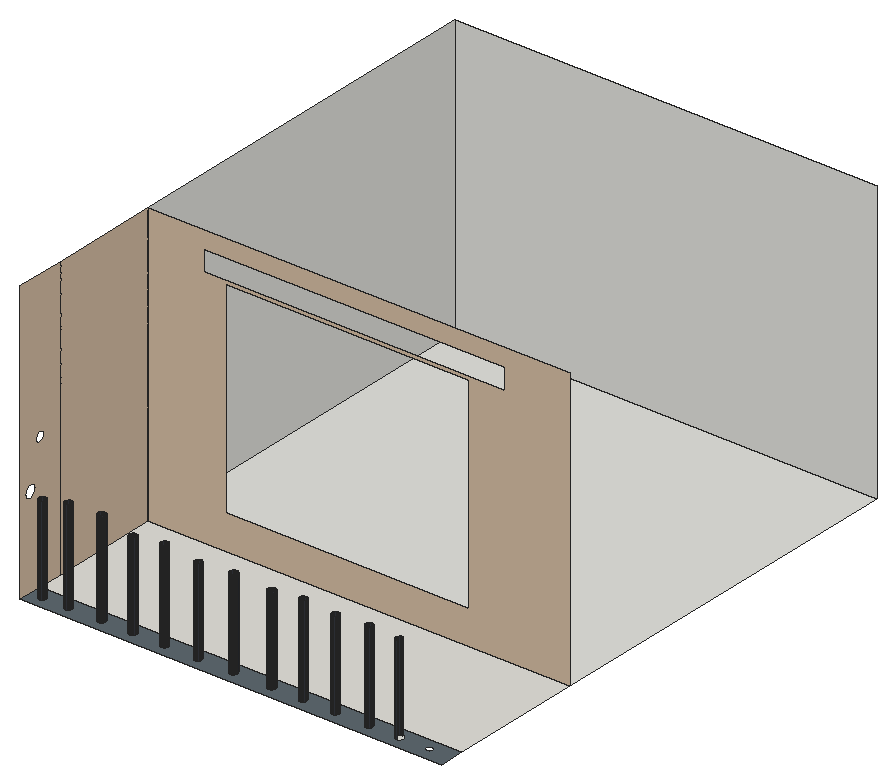
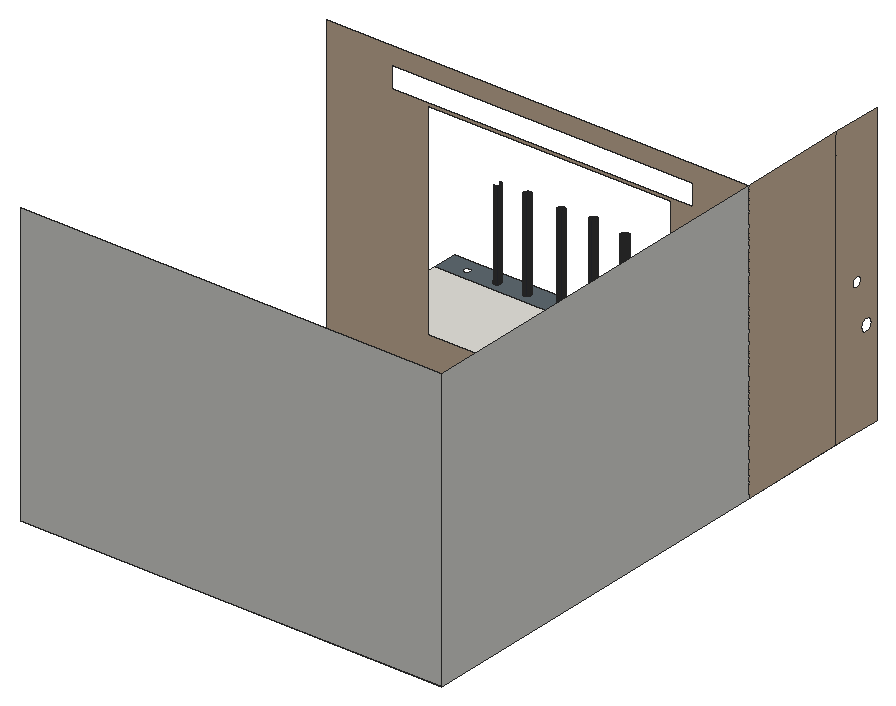
# SketchUp Ruby script. Lengths in inches.
U = 1.inch
M = Sketchup.active_model
def pt(a) = Geom::Point3d.new(a.map { |v| v * U })
def face(e, loops, mat)
  f = e.add_face(loops[0].map { |a| pt(a) })
  loops[1..].each { |l| e.add_face(l.map { |a| pt(a) }).erase! }
  f.material = f.back_material = mat if mat
  f
end
# faces: each face lists its corners as indices into pts; further lists are holes
def faces(e, pts, list, mat = nil) = list.each { |f| face(e, (f[0].is_a?(Array) ? f : [f]).map { |l| l.map { |i| pts[i] } }, mat) }
# xy, xz, yz: faces in a plane at the given z, y or x. An outline is a flat list of corners, or four numbers for a rectangle; further outlines are holes
def ring(l) = l.size == 4 ? [[l[0], l[1]], [l[2], l[1]], [l[2], l[3]], [l[0], l[3]]] : l.each_slice(2).to_a
def flat(e, list, mat, &to3) = list.each { |f| face(e, (f[0].is_a?(Array) ? f : [f]).map { |l| ring(l).map { |u, v| to3.(u, v) } }, mat) }
def xy(e, z, list, mat = nil) = flat(e, list, mat) { |x, y| [x, y, z] }
def xz(e, y, list, mat = nil) = flat(e, list, mat) { |x, z| [x, y, z] }
def yz(e, x, list, mat = nil) = flat(e, list, mat) { |y, z| [x, y, z] }
def lines(e, pts, list) = list.each { |a, b| e.add_line(pt(pts[a]), pt(pts[b])) }
# prism: a flat outline (further loops are holes) pulled along v
def prism(e, loops, v, mat = nil)
  f = face(e, loops, mat); d = Geom::Vector3d.new(v.map { |x| x * U })
  f.pushpull(f.normal.samedirection?(d) ? d.length : -d.length)
end
def box(e, o, s, mat = nil) = prism(e, [[o, [o[0] + s[0], o[1], o[2]], [o[0] + s[0], o[1] + s[1], o[2]], [o[0], o[1] + s[1], o[2]]]], [0, 0, s[2]], mat)
def at(x, y, z, deg = 0) = Geom::Transformation.translation(pt([x, y, z])) * Geom::Transformation.rotation(ORIGIN, Z_AXIS, deg.degrees)
def axes(o, x, y, z) = Geom::Transformation.new([*x, 0, *y, 0, *z, 0, *pt(o).to_a, 1])
def part(name) = M.definitions.add(name)
# library, detail: a bought-in or finely detailed component or shape, given as its bounding box
def library(name, o, s) = part(name).tap { |d| box(d.entities, o, s) }
def detail(e, o, s) = box(e.add_group.entities, o, s)
def put(e, d, t, mat = nil) = e.add_instance(d, t).tap { |i| i.material = mat if mat }
def group(e, t, mat = nil) = e.add_group.tap { |g| g.transformation = t; g.material = mat if mat }.entities
root = M.entities
M.materials.add("[Formica Laminate Dark]").color = [50, 53, 60]
M.materials.add("[Formica Laminate Light]").color = [213, 189, 164]
M.materials.add("[Formica Speckled Grey]").color = [94, 105, 111]
M.materials.add("[Marble Carrara Gold Floor Tile]").color = [225, 223, 217]
xy(root,381,[[13.88,126.78,13.48,126.87,13.125,127.0625,12.83,127.34,12.61,127.6875,12.49,128.08,12.48,128.48,12.57,128.88,12.76,129.24,13.04,129.54,13.39,129.76,13.78,129.875,14.18,129.89,14.58,129.8,14.94,129.6,15.24,129.33,15.46,128.98,15.57,128.59,15.59,128.18,15.5,127.78,15.3,127.42,15.03,127.125,14.68,126.91,14.29,126.79],[25.07,126.78,24.67,126.87,24.3125,127.0625,24.01,127.34,23.8,127.6875,23.68,128.08,23.67,128.48,23.76,128.88,23.95,129.24,24.23,129.54,24.57,129.76,24.96,129.875,25.37,129.89,25.77,129.8,26.13,129.6,26.43,129.33,26.64,128.98,26.76,128.59,26.78,128.18,26.68,127.78,26.49,127.42,26.21,127.125,25.87,126.91,25.48,126.79],[39.26,126.78,38.86,126.87,38.5,127.0625,38.2,127.34,37.99,127.6875,37.87,128.08,37.85,128.48,37.94,128.88,38.14,129.24,38.42,129.54,38.76,129.76,39.15,129.875,39.56,129.89,39.96,129.8,40.32,129.6,40.61,129.33,40.83,128.98,40.95,128.59,40.96,128.18,40.87,127.78,40.68,127.42,40.4,127.125,40.05,126.91,39.66,126.79],[52.63,126.78,52.23,126.87,51.875,127.0625,51.58,127.34,51.36,127.6875,51.24,128.08,51.23,128.48,51.32,128.88,51.51,129.24,51.79,129.54,52.14,129.76,52.53,129.875,52.93,129.89,53.33,129.8,53.69,129.6,53.99,129.33,54.21,128.98,54.32,128.59,54.34,128.18,54.25,127.78,54.05,127.42,53.78,127.125,53.43,126.91,53.04,126.79],[66.19,126.78,65.8,126.87,65.4375,127.0625,65.14,127.34,64.92,127.6875,64.8,128.08,64.79,128.48,64.88,128.88,65.07,129.24,65.35,129.54,65.7,129.76,66.09,129.875,66.5,129.89,66.89,129.8,67.25,129.6,67.55,129.33,67.77,128.98,67.89,128.59,67.9,128.18,67.81,127.78,67.62,127.42,67.34,127.125,66.99,126.91,66.6,126.79],
  [80.57,126.78,80.17,126.87,79.8125,127.0625,79.51,127.34,79.3,127.6875,79.18,128.08,79.17,128.48,79.26,128.88,79.45,129.24,79.73,129.54,80.07,129.76,80.46,129.875,80.87,129.89,81.27,129.8,81.63,129.6,81.93,129.33,82.14,128.98,82.26,128.59,82.28,128.18,82.18,127.78,81.99,127.42,81.71,127.125,81.37,126.91,80.98,126.79],[95.76,126.78,95.36,126.87,95,127.0625,94.7,127.34,94.49,127.6875,94.37,128.08,94.35,128.48,94.44,128.88,94.64,129.24,94.92,129.54,95.26,129.76,95.65,129.875,96.06,129.89,96.46,129.8,96.82,129.6,97.11,129.33,97.33,128.98,97.45,128.59,97.46,128.18,97.37,127.78,97.18,127.42,96.9,127.125,96.55,126.91,96.16,126.79],[112.07,126.78,111.67,126.87,111.3125,127.0625,111.01,127.34,110.8,127.6875,110.68,128.08,110.67,128.48,110.76,128.88,110.95,129.24,111.23,129.54,111.57,129.76,111.96,129.875,112.37,129.89,112.77,129.8,113.13,129.6,113.43,129.33,113.64,128.98,113.76,128.59,113.78,128.18,113.68,127.78,113.49,127.42,113.21,127.125,112.87,126.91,112.48,126.79],[125.44,126.78,125.05,126.87,124.6875,127.0625,124.39,127.34,124.17,127.6875,124.05,128.08,124.04,128.48,124.13,128.88,124.32,129.24,124.6,129.54,124.95,129.76,125.34,129.875,125.75,129.89,126.14,129.8,126.5,129.6,126.8,129.33,127.02,128.98,127.14,128.59,127.15,128.18,127.06,127.78,126.87,127.42,126.59,127.125,126.24,126.91,125.85,126.79],[139.32,126.78,138.92,126.87,138.5625,127.0625,138.26,127.34,138.05,127.6875,137.93,128.08,137.92,128.48,138.01,128.88,138.2,129.24,138.48,129.54,138.82,129.76,139.21,129.875,139.62,129.89,140.02,129.8,140.38,129.6,140.68,129.33,140.89,128.98,141.01,128.59,141.03,128.18,140.93,127.78,140.74,127.42,140.46,127.125,140.12,126.91,139.73,126.79],
  [153.76,126.78,153.36,126.87,153,127.0625,152.7,127.34,152.49,127.6875,152.37,128.08,152.35,128.48,152.44,128.88,152.64,129.24,152.92,129.54,153.26,129.76,153.65,129.875,154.06,129.89,154.46,129.8,154.82,129.6,155.11,129.33,155.33,128.98,155.45,128.59,155.46,128.18,155.37,127.78,155.18,127.42,154.9,127.125,154.55,126.91,154.16,126.79],[166.69,126.78,166.3,126.87,165.9375,127.0625,165.64,127.34,165.42,127.6875,165.3,128.08,165.29,128.48,165.38,128.88,165.57,129.24,165.85,129.54,166.2,129.76,166.59,129.875,167,129.89,167.39,129.8,167.75,129.6,168.05,129.33,168.27,128.98,168.39,128.59,168.4,128.18,168.31,127.78,168.12,127.42,167.84,127.125,167.49,126.91,167.1,126.79],[9,191.15,189.57,355.125]])
xy(root,381,[[[9,122.79,189.57,133.5],[179.57,126.78,179.17,126.87,178.8125,127.0625,178.51,127.34,178.3,127.6875,178.18,128.08,178.17,128.48,178.26,128.88,178.45,129.24,178.73,129.54,179.07,129.76,179.46,129.875,179.87,129.89,180.27,129.8,180.63,129.6,180.93,129.33,181.14,128.98,181.26,128.59,181.28,128.18,181.18,127.78,180.99,127.42,180.71,127.125,180.37,126.91,179.98,126.79],[13.88,126.78,13.48,126.87,13.125,127.0625,12.83,127.34,12.61,127.6875,12.49,128.08,12.48,128.48,12.57,128.88,12.76,129.24,13.04,129.54,13.39,129.76,13.78,129.875,14.18,129.89,14.58,129.8,14.94,129.6,15.24,129.33,15.46,128.98,15.57,128.59,15.59,128.18,15.5,127.78,15.3,127.42,15.03,127.125,14.68,126.91,14.29,126.79],[166.69,126.78,166.3,126.87,165.9375,127.0625,165.64,127.34,165.42,127.6875,165.3,128.08,165.29,128.48,165.38,128.88,165.57,129.24,165.85,129.54,166.2,129.76,166.59,129.875,167,129.89,167.39,129.8,167.75,129.6,168.05,129.33,168.27,128.98,168.39,128.59,168.4,128.18,168.31,127.78,168.12,127.42,167.84,127.125,167.49,126.91,167.1,126.79],[25.07,126.78,24.67,126.87,24.3125,127.0625,24.01,127.34,23.8,127.6875,23.68,128.08,23.67,128.48,23.76,128.88,23.95,129.24,24.23,129.54,24.57,129.76,24.96,129.875,25.37,129.89,25.77,129.8,26.13,129.6,26.43,129.33,26.64,128.98,26.76,128.59,26.78,128.18,26.68,127.78,26.49,127.42,26.21,127.125,25.87,126.91,25.48,126.79],[153.76,126.78,153.36,126.87,153,127.0625,152.7,127.34,152.49,127.6875,152.37,128.08,152.35,128.48,152.44,128.88,152.64,129.24,152.92,129.54,153.26,129.76,153.65,129.875,154.06,129.89,154.46,129.8,154.82,129.6,155.11,129.33,155.33,128.98,155.45,128.59,155.46,128.18,155.37,127.78,155.18,127.42,154.9,127.125,154.55,126.91,154.16,126.79],[39.26,126.78,38.86,126.87,38.5,127.0625,38.2,127.34,37.99,127.6875,37.87,128.08,37.85,128.48,37.94,128.88,38.14,129.24,38.42,129.54,38.76,129.76,39.15,129.875,39.56,129.89,39.96,129.8,40.32,129.6,40.61,129.33,40.83,128.98,40.95,128.59,40.96,128.18,40.87,127.78,40.68,127.42,40.4,127.125,40.05,126.91,39.66,126.79],[139.32,126.78,138.92,126.87,138.5625,127.0625,138.26,127.34,138.05,127.6875,137.93,128.08,137.92,128.48,138.01,128.88,138.2,129.24,138.48,129.54,138.82,129.76,139.21,129.875,139.62,129.89,140.02,129.8,140.38,129.6,140.68,129.33,140.89,128.98,141.01,128.59,141.03,128.18,140.93,127.78,140.74,127.42,140.46,127.125,140.12,126.91,139.73,126.79],[52.63,126.78,52.23,126.87,51.875,127.0625,51.58,127.34,51.36,127.6875,51.24,128.08,51.23,128.48,51.32,128.88,51.51,129.24,51.79,129.54,52.14,129.76,52.53,129.875,52.93,129.89,53.33,129.8,53.69,129.6,53.99,129.33,54.21,128.98,54.32,128.59,54.34,128.18,54.25,127.78,54.05,127.42,53.78,127.125,53.43,126.91,53.04,126.79],[125.44,126.78,125.05,126.87,124.6875,127.0625,124.39,127.34,124.17,127.6875,124.05,128.08,124.04,128.48,124.13,128.88,124.32,129.24,124.6,129.54,124.95,129.76,125.34,129.875,125.75,129.89,126.14,129.8,126.5,129.6,126.8,129.33,127.02,128.98,127.14,128.59,127.15,128.18,127.06,127.78,126.87,127.42,126.59,127.125,126.24,126.91,125.85,126.79],[66.19,126.78,65.8,126.87,65.4375,127.0625,65.14,127.34,64.92,127.6875,64.8,128.08,64.79,128.48,64.88,128.88,65.07,129.24,65.35,129.54,65.7,129.76,66.09,129.875,66.5,129.89,66.89,129.8,67.25,129.6,67.55,129.33,67.77,128.98,67.89,128.59,67.9,128.18,67.81,127.78,67.62,127.42,67.34,127.125,66.99,126.91,66.6,126.79],[112.07,126.78,111.67,126.87,111.3125,127.0625,111.01,127.34,110.8,127.6875,110.68,128.08,110.67,128.48,110.76,128.88,110.95,129.24,111.23,129.54,111.57,129.76,111.96,129.875,112.37,129.89,112.77,129.8,113.13,129.6,113.43,129.33,113.64,128.98,113.76,128.59,113.78,128.18,113.68,127.78,113.49,127.42,113.21,127.125,112.87,126.91,112.48,126.79],[80.57,126.78,80.17,126.87,79.8125,127.0625,79.51,127.34,79.3,127.6875,79.18,128.08,79.17,128.48,79.26,128.88,79.45,129.24,79.73,129.54,80.07,129.76,80.46,129.875,80.87,129.89,81.27,129.8,81.63,129.6,81.93,129.33,82.14,128.98,82.26,128.59,82.28,128.18,82.18,127.78,81.99,127.42,81.71,127.125,81.37,126.91,80.98,126.79],[95.76,126.78,95.36,126.87,95,127.0625,94.7,127.34,94.49,127.6875,94.37,128.08,94.35,128.48,94.44,128.88,94.64,129.24,94.92,129.54,95.26,129.76,95.65,129.875,96.06,129.89,96.46,129.8,96.82,129.6,97.11,129.33,97.33,128.98,97.45,128.59,97.46,128.18,97.37,127.78,97.18,127.42,96.9,127.125,96.55,126.91,96.16,126.79]]],"[Formica Speckled Grey]")
xy(root,381,[[9,133.5,189.57,191.15]],"[Marble Carrara Gold Floor Tile]")
xz(root,191.15,[[[9,381,189.57,501],[42.1875,395.58,146.3125,483.45],[32.67,484.63,161.92,493.63]]],"[Formica Laminate Light]")
xz(root,355.125,[[9,381,189.57,501]])
yz(root,9,[[191.15,381,355.125,501]])
yz(root,9,[[[122.79,381,144.21,501],[128.15,417.26,127.45,417.35,126.8,417.625,126.25,418.05,125.82,418.61,125.55,419.26,125.46,419.95,125.55,420.65,125.82,421.29,126.25,421.85,126.8,422.28,127.45,422.55,128.15,422.64,128.84,422.55,129.49,422.28,130.05,421.85,130.48,421.29,130.74,420.65,130.84,419.95,130.74,419.26,130.48,418.61,130.05,418.05,129.49,417.625,128.84,417.35],[133.36,436.53,132.81,436.61,132.3,436.82,131.86,437.16,131.52,437.6,131.31,438.11,131.23,438.66,131.31,439.21,131.52,439.72,131.86,440.16,132.3,440.5,132.81,440.71,133.36,440.78,133.91,440.71,134.42,440.5,134.86,440.16,135.2,439.72,135.41,439.21,135.48,438.66,135.41,438.11,135.2,437.6,134.86,437.16,134.42,436.82,133.91,436.61]],[144.21,381,191.15,501]],"[Formica Laminate Light]")
p = [[13.48,126.87,381],[13.88,126.78,381],[13.88,126.78,418.625],[13.48,126.87,418.625],[14.29,126.79,381],[14.29,126.79,418.625],
  [14.68,126.91,381],[14.68,126.91,418.625],[24.67,126.87,381],[25.07,126.78,381],[25.07,126.78,421.29],[24.67,126.87,421.29],
  [25.48,126.79,381],[25.48,126.79,421.29],[25.87,126.91,381],[25.87,126.91,421.29],[38.86,126.87,381],[39.26,126.78,381],
  [39.26,126.78,421.85],[38.86,126.87,421.85],[39.66,126.79,381],[39.66,126.79,421.85],[40.05,126.91,381],[40.05,126.91,421.85],
  [52.23,126.87,381],[52.63,126.78,381],[52.63,126.78,418.3125],[52.23,126.87,418.3125],[53.04,126.79,381],[53.04,126.79,418.3125],
  [53.43,126.91,381],[53.43,126.91,418.3125],[65.8,126.87,381],[66.19,126.78,381],[66.19,126.78,420.0625],[65.8,126.87,420.0625],
  [66.6,126.79,381],[66.6,126.79,420.0625],[66.99,126.91,381],[66.99,126.91,420.0625],[80.17,126.87,381],[80.57,126.78,381],
  [80.57,126.78,418],[80.17,126.87,418],[80.98,126.79,381],[80.98,126.79,418],[81.37,126.91,381],[81.37,126.91,418],
  [95.36,126.87,381],[95.76,126.78,381],[95.76,126.78,419.3125],[95.36,126.87,419.3125],[96.16,126.79,381],[96.16,126.79,419.3125],
  [96.55,126.91,381],[96.55,126.91,419.3125],[111.67,126.87,381],[112.07,126.78,381],[112.07,126.78,418.375],[111.67,126.87,418.375],
  [112.48,126.79,381],[112.48,126.79,418.375],[112.87,126.91,381],[112.87,126.91,418.375],[125.05,126.87,381],[125.44,126.78,381],
  [125.44,126.78,419.75],[125.05,126.87,419.75],[125.85,126.79,381],[125.85,126.79,419.75],[126.24,126.91,381],[126.24,126.91,419.75],
  [138.92,126.87,381],[139.32,126.78,381],[139.32,126.78,418.5625],[138.92,126.87,418.5625],[139.73,126.79,381],[139.73,126.79,418.5625],
  [140.12,126.91,381],[140.12,126.91,418.5625],[153.36,126.87,381],[153.76,126.78,381],[153.76,126.78,419.5],[153.36,126.87,419.5],
  [154.16,126.79,381],[154.16,126.79,419.5],[154.55,126.91,381],[154.55,126.91,419.5],[166.3,126.87,381],[166.69,126.78,381],
  [166.69,126.78,418.875],[166.3,126.87,418.875],[167.1,126.79,381],[167.1,126.79,418.875],[13.125,127.0625,381],[13.125,127.0625,418.625],
  [15.03,127.125,381],[15.03,127.125,418.625],[24.3125,127.0625,381],[24.3125,127.0625,421.29],[26.21,127.125,381],[26.21,127.125,421.29],
  [38.5,127.0625,381],[38.5,127.0625,421.85],[40.4,127.125,381],[40.4,127.125,421.85],[51.875,127.0625,381],[51.875,127.0625,418.3125],
  [53.78,127.125,381],[53.78,127.125,418.3125],[65.4375,127.0625,381],[65.4375,127.0625,420.0625],[67.34,127.125,381],[67.34,127.125,420.0625],
  [79.8125,127.0625,381],[79.8125,127.0625,418],[81.71,127.125,381],[81.71,127.125,418],[95,127.0625,381],[95,127.0625,419.3125],
  [96.9,127.125,381],[96.9,127.125,419.3125],[111.3125,127.0625,381],[111.3125,127.0625,418.375],[113.21,127.125,381],[113.21,127.125,418.375],
  [124.6875,127.0625,381],[124.6875,127.0625,419.75],[126.59,127.125,381],[126.59,127.125,419.75],[138.5625,127.0625,381],[138.5625,127.0625,418.5625],
  [140.46,127.125,381],[140.46,127.125,418.5625],[153,127.0625,381],[153,127.0625,419.5],[154.9,127.125,381],[154.9,127.125,419.5],
  [165.9375,127.0625,381],[165.9375,127.0625,418.875],[12.83,127.34,381],[12.83,127.34,418.625],[15.3,127.42,381],[15.3,127.42,418.625],
  [24.01,127.34,381],[24.01,127.34,421.29],[26.49,127.42,381],[26.49,127.42,421.29],[38.2,127.34,381],[38.2,127.34,421.85],
  [40.68,127.42,381],[40.68,127.42,421.85],[51.58,127.34,381],[51.58,127.34,418.3125],[54.05,127.42,381],[54.05,127.42,418.3125],
  [65.14,127.34,381],[65.14,127.34,420.0625],[67.62,127.42,381],[67.62,127.42,420.0625],[79.51,127.34,381],[79.51,127.34,418],
  [81.99,127.42,381],[81.99,127.42,418],[94.7,127.34,381],[94.7,127.34,419.3125],[97.18,127.42,381],[97.18,127.42,419.3125],
  [111.01,127.34,381],[111.01,127.34,418.375],[113.49,127.42,381],[113.49,127.42,418.375],[124.39,127.34,381],[124.39,127.34,419.75],
  [126.87,127.42,381],[126.87,127.42,419.75],[138.26,127.34,381],[138.26,127.34,418.5625],[140.74,127.42,381],[140.74,127.42,418.5625],
  [152.7,127.34,381],[152.7,127.34,419.5],[155.18,127.42,381],[155.18,127.42,419.5],[165.64,127.34,381],[165.64,127.34,418.875],
  [12.61,127.6875,381],[12.61,127.6875,418.625],[23.8,127.6875,381],[23.8,127.6875,421.29],[37.99,127.6875,381],[37.99,127.6875,421.85],
  [51.36,127.6875,381],[51.36,127.6875,418.3125],[64.92,127.6875,381],[64.92,127.6875,420.0625],[79.3,127.6875,381],[79.3,127.6875,418],
  [94.49,127.6875,381],[94.49,127.6875,419.3125],[110.8,127.6875,381],[110.8,127.6875,418.375],[124.17,127.6875,381],[124.17,127.6875,419.75],
  [138.05,127.6875,381],[138.05,127.6875,418.5625],[152.49,127.6875,381],[152.49,127.6875,419.5],[165.42,127.6875,381],[165.42,127.6875,418.875],
  [15.5,127.78,381],[15.5,127.78,418.625],[26.68,127.78,381],[26.68,127.78,421.29],[40.87,127.78,381],[40.87,127.78,421.85],
  [54.25,127.78,381],[54.25,127.78,418.3125],[67.81,127.78,381],[67.81,127.78,420.0625],[82.18,127.78,381],[82.18,127.78,418],
  [97.37,127.78,381],[97.37,127.78,419.3125],[113.68,127.78,381],[113.68,127.78,418.375],[127.06,127.78,381],[127.06,127.78,419.75],
  [140.93,127.78,381],[140.93,127.78,418.5625],[155.37,127.78,381],[155.37,127.78,419.5],[12.49,128.08,381],[12.49,128.08,418.625],
  [23.68,128.08,381],[23.68,128.08,421.29],[37.87,128.08,381],[37.87,128.08,421.85],[51.24,128.08,381],[51.24,128.08,418.3125],
  [64.8,128.08,381],[64.8,128.08,420.0625],[79.18,128.08,381],[79.18,128.08,418],[94.37,128.08,381],[94.37,128.08,419.3125],
  [110.68,128.08,381],[110.68,128.08,418.375],[124.05,128.08,381],[124.05,128.08,419.75],[137.93,128.08,381],[137.93,128.08,418.5625],
  [152.37,128.08,381],[152.37,128.08,419.5],[165.3,128.08,381],[165.3,128.08,418.875],[15.59,128.18,381],[15.59,128.18,418.625],
  [26.78,128.18,381],[26.78,128.18,421.29],[40.96,128.18,381],[40.96,128.18,421.85],[54.34,128.18,381],[54.34,128.18,418.3125],
  [67.9,128.18,381],[67.9,128.18,420.0625],[82.28,128.18,381],[82.28,128.18,418],[97.46,128.18,381],[97.46,128.18,419.3125],
  [113.78,128.18,381],[113.78,128.18,418.375],[127.15,128.18,381],[127.15,128.18,419.75],[141.03,128.18,381],[141.03,128.18,418.5625],
  [155.46,128.18,381],[155.46,128.18,419.5],[12.48,128.48,381],[12.48,128.48,418.625],[23.67,128.48,381],[23.67,128.48,421.29],
  [37.85,128.48,381],[37.85,128.48,421.85],[51.23,128.48,381],[51.23,128.48,418.3125],[64.79,128.48,381],[64.79,128.48,420.0625],
  [79.17,128.48,381],[79.17,128.48,418],[94.35,128.48,381],[94.35,128.48,419.3125],[110.67,128.48,381],[110.67,128.48,418.375],
  [124.04,128.48,381],[124.04,128.48,419.75],[137.92,128.48,381],[137.92,128.48,418.5625],[152.35,128.48,381],[152.35,128.48,419.5],
  [165.29,128.48,381],[165.29,128.48,418.875],[15.57,128.59,381],[15.57,128.59,418.625],[26.76,128.59,381],[26.76,128.59,421.29],
  [40.95,128.59,381],[40.95,128.59,421.85],[54.32,128.59,381],[54.32,128.59,418.3125],[67.89,128.59,381],[67.89,128.59,420.0625],
  [82.26,128.59,381],[82.26,128.59,418],[97.45,128.59,381],[97.45,128.59,419.3125],[113.76,128.59,381],[113.76,128.59,418.375],
  [127.14,128.59,381],[127.14,128.59,419.75],[141.01,128.59,381],[141.01,128.59,418.5625],[155.45,128.59,381],[155.45,128.59,419.5],
  [12.57,128.88,381],[12.57,128.88,418.625],[23.76,128.88,381],[23.76,128.88,421.29],[37.94,128.88,381],[37.94,128.88,421.85],
  [51.32,128.88,381],[51.32,128.88,418.3125],[64.88,128.88,381],[64.88,128.88,420.0625],[79.26,128.88,381],[79.26,128.88,418],
  [94.44,128.88,381],[94.44,128.88,419.3125],[110.76,128.88,381],[110.76,128.88,418.375],[124.13,128.88,381],[124.13,128.88,419.75],
  [138.01,128.88,381],[138.01,128.88,418.5625],[152.44,128.88,381],[152.44,128.88,419.5],[165.38,128.88,381],[165.38,128.88,418.875],
  [15.46,128.98,381],[15.46,128.98,418.625],[26.64,128.98,381],[26.64,128.98,421.29],[40.83,128.98,381],[40.83,128.98,421.85],
  [54.21,128.98,381],[54.21,128.98,418.3125],[67.77,128.98,381],[67.77,128.98,420.0625],[82.14,128.98,381],[82.14,128.98,418],
  [97.33,128.98,381],[97.33,128.98,419.3125],[113.64,128.98,381],[113.64,128.98,418.375],[127.02,128.98,381],[127.02,128.98,419.75],
  [140.89,128.98,381],[140.89,128.98,418.5625],[155.33,128.98,381],[155.33,128.98,419.5],[12.76,129.24,381],[12.76,129.24,418.625],
  [23.95,129.24,381],[23.95,129.24,421.29],[38.14,129.24,381],[38.14,129.24,421.85],[51.51,129.24,381],[51.51,129.24,418.3125],
  [65.07,129.24,381],[65.07,129.24,420.0625],[79.45,129.24,381],[79.45,129.24,418],[94.64,129.24,381],[94.64,129.24,419.3125],
  [110.95,129.24,381],[110.95,129.24,418.375],[124.32,129.24,381],[124.32,129.24,419.75],[138.2,129.24,381],[138.2,129.24,418.5625],
  [152.64,129.24,381],[152.64,129.24,419.5],[165.57,129.24,381],[165.57,129.24,418.875],[15.24,129.33,381],[15.24,129.33,418.625],
  [26.43,129.33,381],[26.43,129.33,421.29],[40.61,129.33,381],[40.61,129.33,421.85],[53.99,129.33,381],[53.99,129.33,418.3125],
  [67.55,129.33,381],[67.55,129.33,420.0625],[81.93,129.33,381],[81.93,129.33,418],[97.11,129.33,381],[97.11,129.33,419.3125],
  [113.43,129.33,381],[113.43,129.33,418.375],[126.8,129.33,381],[126.8,129.33,419.75],[140.68,129.33,381],[140.68,129.33,418.5625],
  [155.11,129.33,381],[155.11,129.33,419.5],[13.04,129.54,381],[13.04,129.54,418.625],[24.23,129.54,381],[24.23,129.54,421.29],
  [38.42,129.54,381],[38.42,129.54,421.85],[51.79,129.54,381],[51.79,129.54,418.3125],[65.35,129.54,381],[65.35,129.54,420.0625],
  [79.73,129.54,381],[79.73,129.54,418],[94.92,129.54,381],[94.92,129.54,419.3125],[111.23,129.54,381],[111.23,129.54,418.375],
  [124.6,129.54,381],[124.6,129.54,419.75],[138.48,129.54,381],[138.48,129.54,418.5625],[152.92,129.54,381],[152.92,129.54,419.5],
  [165.85,129.54,381],[165.85,129.54,418.875],[14.94,129.6,381],[14.94,129.6,418.625],[26.13,129.6,381],[26.13,129.6,421.29],
  [40.32,129.6,381],[40.32,129.6,421.85],[53.69,129.6,381],[53.69,129.6,418.3125],[67.25,129.6,381],[67.25,129.6,420.0625],
  [81.63,129.6,381],[81.63,129.6,418],[96.82,129.6,381],[96.82,129.6,419.3125],[113.13,129.6,381],[113.13,129.6,418.375],
  [126.5,129.6,381],[126.5,129.6,419.75],[140.38,129.6,381],[140.38,129.6,418.5625],[154.82,129.6,381],[154.82,129.6,419.5],
  [13.39,129.76,381],[13.39,129.76,418.625],[24.57,129.76,381],[24.57,129.76,421.29],[38.76,129.76,381],[38.76,129.76,421.85],
  [52.14,129.76,381],[52.14,129.76,418.3125],[65.7,129.76,381],[65.7,129.76,420.0625],[80.07,129.76,381],[80.07,129.76,418],
  [95.26,129.76,381],[95.26,129.76,419.3125],[111.57,129.76,381],[111.57,129.76,418.375],[124.95,129.76,381],[124.95,129.76,419.75],
  [138.82,129.76,381],[138.82,129.76,418.5625],[153.26,129.76,381],[153.26,129.76,419.5],[166.2,129.76,381],[166.2,129.76,418.875],
  [14.58,129.8,381],[14.58,129.8,418.625],[25.77,129.8,381],[25.77,129.8,421.29],[39.96,129.8,381],[39.96,129.8,421.85],
  [53.33,129.8,381],[53.33,129.8,418.3125],[66.89,129.8,381],[66.89,129.8,420.0625],[81.27,129.8,381],[81.27,129.8,418],
  [96.46,129.8,381],[96.46,129.8,419.3125],[112.77,129.8,381],[112.77,129.8,418.375],[126.14,129.8,381],[126.14,129.8,419.75],
  [140.02,129.8,381],[140.02,129.8,418.5625],[154.46,129.8,381],[154.46,129.8,419.5],[13.78,129.875,381],[13.78,129.875,418.625],
  [14.18,129.89,381],[14.18,129.89,418.625],[24.96,129.875,381],[24.96,129.875,421.29],[25.37,129.89,381],[25.37,129.89,421.29],
  [39.15,129.875,381],[39.15,129.875,421.85],[39.56,129.89,381],[39.56,129.89,421.85],[52.53,129.875,381],[52.53,129.875,418.3125],
  [52.93,129.89,381],[52.93,129.89,418.3125],[66.09,129.875,381],[66.09,129.875,420.0625],[66.5,129.89,381],[66.5,129.89,420.0625],
  [80.46,129.875,381],[80.46,129.875,418],[80.87,129.89,381],[80.87,129.89,418],[95.65,129.875,381],[95.65,129.875,419.3125],
  [96.06,129.89,381],[96.06,129.89,419.3125],[111.96,129.875,381],[111.96,129.875,418.375],[112.37,129.89,381],[112.37,129.89,418.375],
  [125.34,129.875,381],[125.34,129.875,419.75],[125.75,129.89,381],[125.75,129.89,419.75],[139.21,129.875,381],[139.21,129.875,418.5625],
  [139.62,129.89,381],[139.62,129.89,418.5625],[153.65,129.875,381],[153.65,129.875,419.5],[154.06,129.89,381],[154.06,129.89,419.5],
  [166.59,129.875,381],[166.59,129.875,418.875],[167,129.89,381],[167,129.89,418.875]]
faces(root,p,[[0,1,2,3],[1,4,5,2],[4,6,7,5],[8,9,10,11],[9,12,13,10],[12,14,15,13],[16,17,18,19],[17,20,21,18],
  [20,22,23,21],[24,25,26,27],[25,28,29,26],[28,30,31,29],[32,33,34,35],[33,36,37,34],[36,38,39,37],[40,41,42,43],
  [41,44,45,42],[44,46,47,45],[48,49,50,51],[49,52,53,50],[52,54,55,53],[56,57,58,59],[57,60,61,58],[60,62,63,61],
  [64,65,66,67],[65,68,69,66],[68,70,71,69],[72,73,74,75],[73,76,77,74],[76,78,79,77],[80,81,82,83],[81,84,85,82],
  [84,86,87,85],[88,89,90,91],[89,92,93,90],[94,0,3,95],[6,96,97,7],[98,8,11,99],[14,100,101,15],[102,16,19,103],
  [22,104,105,23],[106,24,27,107],[30,108,109,31],[110,32,35,111],[38,112,113,39],[114,40,43,115],[46,116,117,47],[118,48,51,119],
  [54,120,121,55],[122,56,59,123],[62,124,125,63],[126,64,67,127],[70,128,129,71],[130,72,75,131],[78,132,133,79],[134,80,83,135],
  [86,136,137,87],[138,88,91,139],[140,94,95,141],[96,142,143,97],[144,98,99,145],[100,146,147,101],[148,102,103,149],[104,150,151,105],
  [152,106,107,153],[108,154,155,109],[156,110,111,157],[112,158,159,113],[160,114,115,161],[116,162,163,117],[164,118,119,165],[120,166,167,121],
  [168,122,123,169],[124,170,171,125],[172,126,127,173],[128,174,175,129],[176,130,131,177],[132,178,179,133],[180,134,135,181],[136,182,183,137],
  [184,138,139,185],[186,140,141,187],[188,144,145,189],[190,148,149,191],[192,152,153,193],[194,156,157,195],[196,160,161,197],[198,164,165,199],
  [200,168,169,201],[202,172,173,203],[204,176,177,205],[206,180,181,207],[208,184,185,209],[142,210,211,143],[146,212,213,147],[150,214,215,151],
  [154,216,217,155],[158,218,219,159],[162,220,221,163],[166,222,223,167],[170,224,225,171],[174,226,227,175],[178,228,229,179],[182,230,231,183],
  [232,186,187,233],[234,188,189,235],[236,190,191,237],[238,192,193,239],[240,194,195,241],[242,196,197,243],[244,198,199,245],[246,200,201,247],
  [248,202,203,249],[250,204,205,251],[252,206,207,253],[254,208,209,255],[210,256,257,211],[212,258,259,213],[214,260,261,215],[216,262,263,217],
  [218,264,265,219],[220,266,267,221],[222,268,269,223],[224,270,271,225],[226,272,273,227],[228,274,275,229],[230,276,277,231],[278,232,233,279],
  [280,234,235,281],[282,236,237,283],[284,238,239,285],[286,240,241,287],[288,242,243,289],[290,244,245,291],[292,246,247,293],[294,248,249,295],
  [296,250,251,297],[298,252,253,299],[300,254,255,301],[256,302,303,257],[258,304,305,259],[260,306,307,261],[262,308,309,263],[264,310,311,265],
  [266,312,313,267],[268,314,315,269],[270,316,317,271],[272,318,319,273],[274,320,321,275],[276,322,323,277],[324,278,279,325],[326,280,281,327],
  [328,282,283,329],[330,284,285,331],[332,286,287,333],[334,288,289,335],[336,290,291,337],[338,292,293,339],[340,294,295,341],[342,296,297,343],
  [344,298,299,345],[346,300,301,347],[302,348,349,303],[304,350,351,305],[306,352,353,307],[308,354,355,309],[310,356,357,311],[312,358,359,313],
  [314,360,361,315],[316,362,363,317],[318,364,365,319],[320,366,367,321],[322,368,369,323],[370,324,325,371],[372,326,327,373],[374,328,329,375],
  [376,330,331,377],[378,332,333,379],[380,334,335,381],[382,336,337,383],[384,338,339,385],[386,340,341,387],[388,342,343,389],[390,344,345,391],
  [392,346,347,393],[348,394,395,349],[350,396,397,351],[352,398,399,353],[354,400,401,355],[356,402,403,357],[358,404,405,359],[360,406,407,361],
  [362,408,409,363],[364,410,411,365],[366,412,413,367],[368,414,415,369],[416,370,371,417],[418,372,373,419],[420,374,375,421],[422,376,377,423],
  [424,378,379,425],[426,380,381,427],[428,382,383,429],[430,384,385,431],[432,386,387,433],[434,388,389,435],[436,390,391,437],[438,392,393,439],
  [394,440,441,395],[396,442,443,397],[398,444,445,399],[400,446,447,401],[402,448,449,403],[404,450,451,405],[406,452,453,407],[408,454,455,409],
  [410,456,457,411],[412,458,459,413],[414,460,461,415],[462,416,417,463],[464,418,419,465],[466,420,421,467],[468,422,423,469],[470,424,425,471],
  [472,426,427,473],[474,428,429,475],[476,430,431,477],[478,432,433,479],[480,434,435,481],[482,436,437,483],[484,438,439,485],[440,486,487,441],
  [442,488,489,443],[444,490,491,445],[446,492,493,447],[448,494,495,449],[450,496,497,451],[452,498,499,453],[454,500,501,455],[456,502,503,457],
  [458,504,505,459],[460,506,507,461],[508,462,463,509],[486,510,511,487],[512,464,465,513],[488,514,515,489],[516,466,467,517],[490,518,519,491],
  [520,468,469,521],[492,522,523,493],[524,470,471,525],[494,526,527,495],[528,472,473,529],[496,530,531,497],[532,474,475,533],[498,534,535,499],
  [536,476,477,537],[500,538,539,501],[540,478,479,541],[502,542,543,503],[544,480,481,545],[504,546,547,505],[548,482,483,549],[506,550,551,507],
  [552,484,485,553],[510,508,509,511],[514,512,513,515],[518,516,517,519],[522,520,521,523],[526,524,525,527],[530,528,529,531],[534,532,533,535],
  [538,536,537,539],[542,540,541,543],[546,544,545,547],[550,548,549,551],[554,552,553,555]],"[Formica Laminate Dark]")
